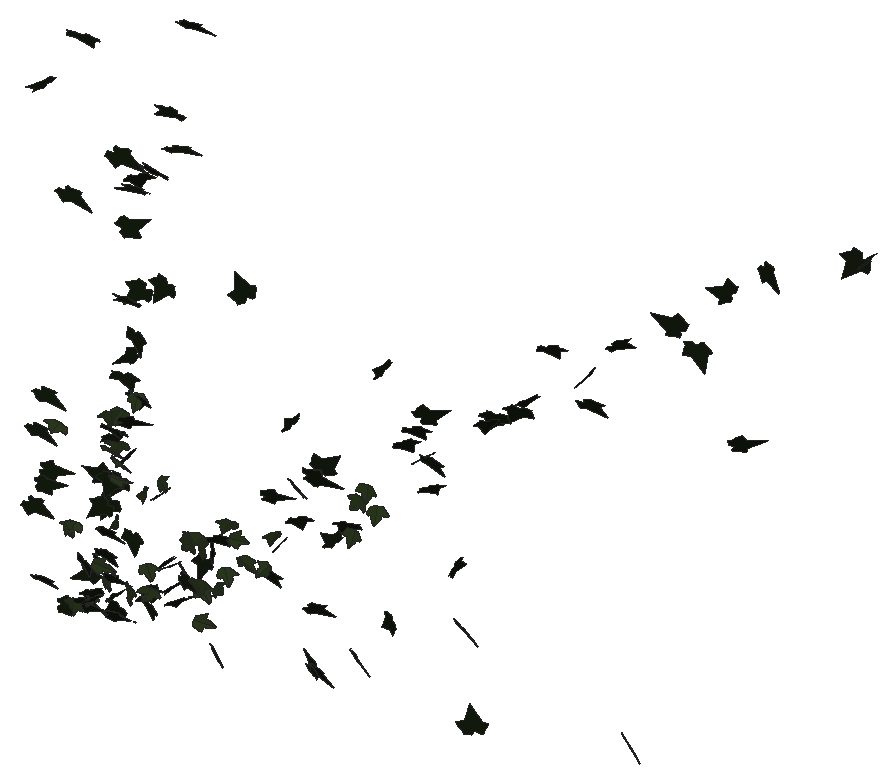
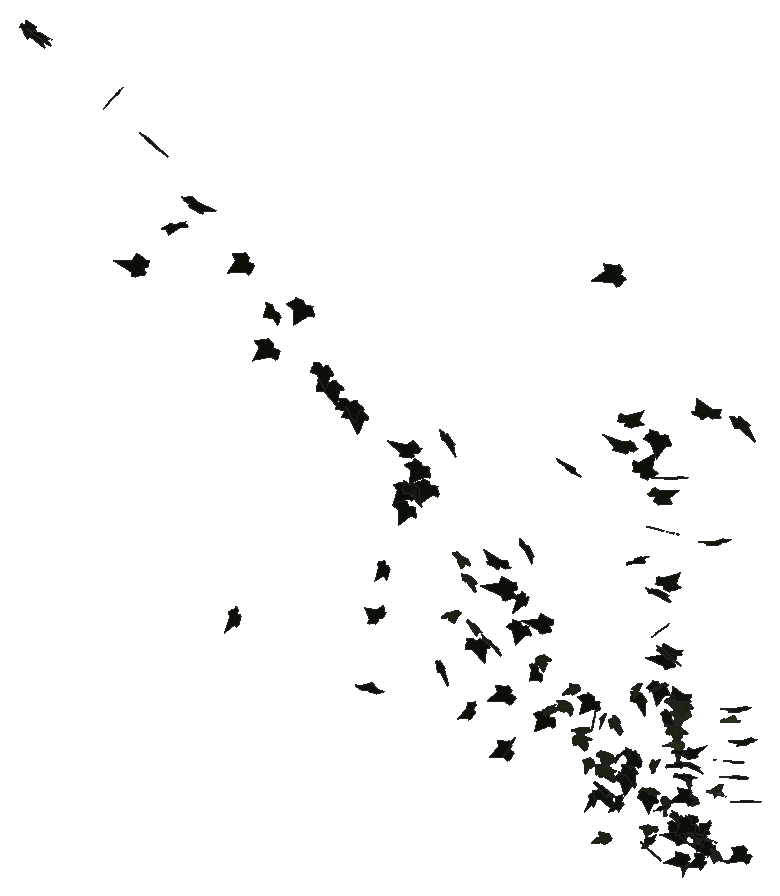
# SketchUp Ruby script. Lengths in inches.
U = 1.inch
M = Sketchup.active_model
def pt(a) = Geom::Point3d.new(a.map { |v| v * U })
def face(e, loops, mat)
  f = e.add_face(loops[0].map { |a| pt(a) })
  loops[1..].each { |l| e.add_face(l.map { |a| pt(a) }).erase! }
  f.material = f.back_material = mat if mat
  f
end
# faces: each face lists its corners as indices into pts; further lists are holes
def faces(e, pts, list, mat = nil) = list.each { |f| face(e, (f[0].is_a?(Array) ? f : [f]).map { |l| l.map { |i| pts[i] } }, mat) }
# xy, xz, yz: faces in a plane at the given z, y or x. An outline is a flat list of corners, or four numbers for a rectangle; further outlines are holes
def ring(l) = l.size == 4 ? [[l[0], l[1]], [l[2], l[1]], [l[2], l[3]], [l[0], l[3]]] : l.each_slice(2).to_a
def flat(e, list, mat, &to3) = list.each { |f| face(e, (f[0].is_a?(Array) ? f : [f]).map { |l| ring(l).map { |u, v| to3.(u, v) } }, mat) }
def xy(e, z, list, mat = nil) = flat(e, list, mat) { |x, y| [x, y, z] }
def xz(e, y, list, mat = nil) = flat(e, list, mat) { |x, z| [x, y, z] }
def yz(e, x, list, mat = nil) = flat(e, list, mat) { |y, z| [x, y, z] }
def lines(e, pts, list) = list.each { |a, b| e.add_line(pt(pts[a]), pt(pts[b])) }
# prism: a flat outline (further loops are holes) pulled along v
def prism(e, loops, v, mat = nil)
  f = face(e, loops, mat); d = Geom::Vector3d.new(v.map { |x| x * U })
  f.pushpull(f.normal.samedirection?(d) ? d.length : -d.length)
end
def box(e, o, s, mat = nil) = prism(e, [[o, [o[0] + s[0], o[1], o[2]], [o[0] + s[0], o[1] + s[1], o[2]], [o[0], o[1] + s[1], o[2]]]], [0, 0, s[2]], mat)
def at(x, y, z, deg = 0) = Geom::Transformation.translation(pt([x, y, z])) * Geom::Transformation.rotation(ORIGIN, Z_AXIS, deg.degrees)
def axes(o, x, y, z) = Geom::Transformation.new([*x, 0, *y, 0, *z, 0, *pt(o).to_a, 1])
def part(name) = M.definitions.add(name)
# library, detail: a bought-in or finely detailed component or shape, given as its bounding box
def library(name, o, s) = part(name).tap { |d| box(d.entities, o, s) }
def detail(e, o, s) = box(e.add_group.entities, o, s)
def put(e, d, t, mat = nil) = e.add_instance(d, t).tap { |i| i.material = mat if mat }
def group(e, t, mat = nil) = e.add_group.tap { |g| g.transformation = t; g.material = mat if mat }.entities
root = M.entities
M.materials.add("1026 AP 7946 SUNNY SIDE UP").color = [254, 231, 186]
M.materials.add("efeu1").color = [18, 25, 13]
M.materials.add("efeu2").color = [43, 57, 29]
c1 = part("ivyleaf_9")
p = [[1.54,2.16,1.25],[1.36,2.04,1.19],[-0.21,0.99,0.68],[-0.71,1.11,0.82],[-0.85,0.86,0.67],[-0.8,0.17,0.21],
  [-0.9,-0.01,0.1],[-0.67,-0.16,-0.02],[-0.08,-0.08,-0.05],[-0.03,-0.6,-0.4],[0.65,-0.88,-0.66],[0.83,-0.6,-0.49],
  [1.29,-0.42,-0.43],[1.8125,-0.07,-0.26],[1.21,0.44,0.15]]
faces(c1.entities,p,[[0,1,2,3,4,5,6,7,8,9,10,11,12,13,14]],"efeu1")
c2 = part("ivyleaf_10")
p = [[0,0.5,-0.03],[-0.0625,2.02,-0.43],[-0.19,2.01,-0.46],[-0.54,1.05,-0.29],[-0.52,0.625,-0.18],[-0.83,0.76,-0.28],
  [-1.16,0.64,-0.33],[-1.15,0.33,-0.24],[-0.77,-0.39,0.02],[-0.3,-0.51,0.16],[0.04,-0.48,0.23],[-0.02,2.01,-0.4375],
  [-0.06,2.01,-0.43],[0.04,-0.49,0.23],[0.67,-0.49,0.14],[1.38,0.36,-0.2],[1.375,0.51,-0.24],[0.81,0.65,-0.19],
  [0.62,0.59,-0.15],[0.6,1.09,-0.28],[0.5,1.23,-0.31]]
faces(c2.entities,p,[[0,1,2,3,4,5,6,7,8,9,10],[11,12,0,13,14,15,16,17,18,19,20]],"efeu2")
put(root,c1,axes([142.13,213.74,300.73],[0.26757,-0.36179,-0.03573],[0.28317,0.11532,-0.34897],[0.49606,0.12932,0.21848]),"1026 AP 7946 SUNNY SIDE UP")
put(root,c1,axes([142.21,213.26,296.25],[0.25217,-0.28686,-0.20351],[0.26459,0.25293,-0.23814],[0.47785,0.01133,0.23925]),"1026 AP 7946 SUNNY SIDE UP")
put(root,c1,axes([142.55,213.89,303.02],[0.2721,-0.36257,-0.07854],[0.28692,0.15483,-0.3402],[0.50626,0.10712,0.23502]),"1026 AP 7946 SUNNY SIDE UP")
put(root,c1,axes([143.6,212.82,323.1],[-0.30014,0.4161,-0.00083],[-0.15211,-0.04776,-0.45862],[-0.63636,-0.18483,0.11001]),"1026 AP 7946 SUNNY SIDE UP")
put(root,c1,axes([142.91,213.24,297.6875],[0.56697,-0.08892,-0.10895],[0.07634,0.35795,-0.13808],[0.20276,0.11386,0.35665]),"1026 AP 7946 SUNNY SIDE UP")
put(root,c1,axes([143.02,212.92,292.01],[0.57279,0.05558,0.03809],[0.04914,0.03732,-0.37797],[-0.09244,0.36421,0.03512]),"1026 AP 7946 SUNNY SIDE UP")
put(root,c1,axes([143.26,213.28,298.71],[0.52552,-0.15164,-0.13523],[0.16581,0.34939,-0.1381],[0.26723,0.08143,0.35163]),"1026 AP 7946 SUNNY SIDE UP")
put(root,c1,axes([143.35,215,315.34],[0.3006,-0.40103,-0.08401],[0.31703,0.16863,-0.37692],[0.55916,0.11998,0.25887]),"1026 AP 7946 SUNNY SIDE UP")
put(root,c2,axes([143.95,213.52,301.57],[-0.57814,-0.03727,0.14265],[0.09812,-0.3848,0.06166],[0.20337,0.07971,0.37579]),"1026 AP 7946 SUNNY SIDE UP")
put(root,c1,axes([143.67,215.91,324.83],[-0.14503,-0.44357,0.16843],[0.58827,-0.17195,-0.26016],[0.45665,0.08063,0.38864]),"1026 AP 7946 SUNNY SIDE UP")
put(root,c2,axes([145.16,213.34,295.85],[-0.58487,-0.02098,0.02789],[0.0317,-0.37281,-0.01438],[0.04372,-0.01033,0.38354]),"1026 AP 7946 SUNNY SIDE UP")
put(root,c1,axes([144.73,212.91,290.9],[0.482,-0.11848,-0.13664],[0.18023,0.33344,-0.03218],[0.2128,-0.01403,0.33675]),"1026 AP 7946 SUNNY SIDE UP")
put(root,c2,axes([145.17,212.77,296],[0.02609,0.34765,0.15016],[-0.02501,0.14444,-0.35705],[-0.59102,0.00923,0.02174]),"1026 AP 7946 SUNNY SIDE UP")
put(root,c2,axes([145.51,212.9375,291.24],[-0.5409,0.08491,0.02844],[-0.07609,-0.08708,-0.35191],[-0.1177,-0.33389,0.0968]),"1026 AP 7946 SUNNY SIDE UP")
put(root,c2,axes([145.48,215.72,291.48],[-0.0806,0.3404,0.08762],[-0.02401,0.08176,-0.35414],[-0.55045,-0.05341,0.00262]),"1026 AP 7946 SUNNY SIDE UP")
put(root,c1,axes([145.41,213.96,293.37],[0.07728,-0.28574,0.22088],[0.10214,-0.20733,-0.29895],[0.55391,0.0781,0.02431]),"1026 AP 7946 SUNNY SIDE UP")
put(root,c1,axes([146.0625,214.07,292.79],[-0.52562,-0.00777,0.13629],[-0.19892,-0.08855,-0.33509],[0.06227,-0.34845,0.07994]),"1026 AP 7946 SUNNY SIDE UP")
put(root,c1,axes([145.54,214.09,291.15],[0.50262,-0.15057,0.00946],[-0.00118,-0.02509,-0.36338],[0.23727,0.31882,-0.02184]),"1026 AP 7946 SUNNY SIDE UP")
put(root,c1,axes([146.21,214.54,298.73],[-0.06225,0.05881,0.38686],[-0.51416,-0.19713,-0.00487],[0.3037,-0.32168,0.07106]),"1026 AP 7946 SUNNY SIDE UP")
put(root,c1,axes([145.625,215.66,291.73],[0.4648,0.00358,0.20448],[0.31179,0.011,-0.30439],[-0.01432,0.35587,0.00943]),"1026 AP 7946 SUNNY SIDE UP")
put(root,c2,axes([146.38,214.58,296.91],[0.33826,-0.26938,-0.15687],[-0.11986,0.13169,-0.35373],[0.47035,0.22728,0.02268]),"1026 AP 7946 SUNNY SIDE UP")
put(root,c1,axes([146.06,214.69,293.88],[0.56469,0.0455,-0.01392],[-0.01436,-0.03694,-0.37135],[-0.07336,0.35749,-0.03445]),"1026 AP 7946 SUNNY SIDE UP")
put(root,c1,axes([145.88,212.94,291.27],[0.26541,-0.01318,0.32018],[0.46806,-0.09615,-0.17126],[0.14247,0.34043,-0.03382]),"1026 AP 7946 SUNNY SIDE UP")
put(root,c2,axes([146.45,215.02,302.5],[-0.38529,-0.3118,-0.00092],[0.03074,-0.01648,-0.40779],[0.48932,-0.24448,0.02489]),"1026 AP 7946 SUNNY SIDE UP")
put(root,c1,axes([146.08,214.21,293.68],[0.45152,-0.18717,0.12069],[0.14043,-0.07922,-0.35316],[0.31851,0.30026,-0.01538]),"1026 AP 7946 SUNNY SIDE UP")
put(root,c2,axes([146.51,213.33,291.98],[0.11829,0.24906,-0.2537],[-0.12127,-0.23541,-0.26937],[-0.53883,0.10766,0.00493]),"1026 AP 7946 SUNNY SIDE UP")
put(root,c1,axes([146.63,214.72,297.21],[-0.44676,-0.24461,-0.03164],[0.06783,-0.00532,-0.38485],[0.38139,-0.28559,0.03137]),"1026 AP 7946 SUNNY SIDE UP")
put(root,c1,axes([146.72,212.8,291.95],[0.15829,0.33526,0.06533],[0.03271,0.05798,-0.36026],[-0.53497,0.10274,-0.0027]),"1026 AP 7946 SUNNY SIDE UP")
put(root,c1,axes([146.8,212.85,292.49],[0.14779,0.31622,-0.14973],[-0.05778,-0.14256,-0.34065],[-0.54537,0.1008,-0.00448]),"1026 AP 7946 SUNNY SIDE UP")
put(root,c2,axes([146.83,215.21,300.66],[-0.51905,-0.19331,0.07779],[-0.07471,-0.0698,-0.3928],[0.3183,-0.33161,0.03465]),"1026 AP 7946 SUNNY SIDE UP")
put(root,c1,axes([146.71,215.46,298.3],[-0.32785,-0.30649,0.08122],[-0.02057,-0.08805,-0.38041],[0.49788,-0.20546,0.03777]),"1026 AP 7946 SUNNY SIDE UP")
put(root,c1,axes([147.03,213.82,297.5],[-0.57913,-0.08341,0.03255],[-0.02998,-0.05955,-0.38544],[0.13728,-0.36488,0.05316]),"1026 AP 7946 SUNNY SIDE UP")
put(root,c1,axes([146.43,214.26,295.55],[0.55766,0.00088,0.10681],[0.16301,-0.00736,-0.36533],[0.00193,0.36942,-0.00537]),"1026 AP 7946 SUNNY SIDE UP")
put(root,c1,axes([146.89,214.59,298.79],[-0.42628,-0.26742,-0.027],[0.08186,-0.01791,-0.38912],[0.41428,-0.27163,0.0491]),"1026 AP 7946 SUNNY SIDE UP")
put(root,c2,axes([146.98,215.28,302.6],[0.60749,-0.0607,-0.07054],[-0.11257,-0.01786,-0.40194],[0.08896,0.3919,-0.02689]),"1026 AP 7946 SUNNY SIDE UP")
put(root,c1,axes([147.57,215.68,306.33],[-0.5662,0.18275,-0.07188],[0.01148,-0.13552,-0.39932],[-0.30796,-0.34104,0.11728]),"1026 AP 7946 SUNNY SIDE UP")
put(root,c1,axes([146.72,215.1,318.87],[0.36025,-0.35595,-0.19957],[0.30419,0.29,-0.31485],[0.55821,0.07169,0.30038]),"1026 AP 7946 SUNNY SIDE UP")
put(root,c2,axes([147.01,214.03,300.95],[-0.13961,-0.33774,0.1794],[0.59888,-0.07814,0.04299],[-0.00196,0.18103,0.35819]),"1026 AP 7946 SUNNY SIDE UP")
put(root,c1,axes([147.25,214.18,302.17],[-0.15527,-0.32678,0.2033],[0.43444,-0.20322,-0.20354],[0.41641,0.09018,0.28816]),"1026 AP 7946 SUNNY SIDE UP")
put(root,c1,axes([147.65,215.7,303.6875],[0.505,0.09081,-0.22566],[-0.33683,-0.04905,-0.34399],[-0.16164,0.38594,0.0118]),"1026 AP 7946 SUNNY SIDE UP")
put(root,c1,axes([147.29,214.0625,301.91],[-0.14049,-0.37426,-0.09172],[0.60408,-0.08564,-0.02745],[0.00935,-0.09056,0.39495]),"1026 AP 7946 SUNNY SIDE UP")
put(root,c2,axes([147.23,214.26,299.04],[0.39017,-0.29292,-0.00677],[0.46063,0.24816,0.00152],[0.00491,-0.00379,0.39546]),"1026 AP 7946 SUNNY SIDE UP")
put(root,c2,axes([147.23,212.79,294.34],[0.11746,0.09075,0.36258],[0.46144,0.19605,-0.11527],[-0.33587,0.30109,-0.03156]),"1026 AP 7946 SUNNY SIDE UP")
put(root,c1,axes([147.52,215.5625,295.02],[-0.05434,-0.37089,0.0083],[0.00994,-0.01079,-0.38373],[0.58332,-0.03437,0.00731]),"1026 AP 7946 SUNNY SIDE UP")
put(root,c2,axes([147.67,215.69,303.68],[0.30586,0.32762,-0.12208],[-0.07216,-0.11258,-0.39278],[-0.54406,0.19912,-0.01653]),"1026 AP 7946 SUNNY SIDE UP")
put(root,c1,axes([147.4375,214.87,314.5625],[0.68626,-0.00428,-0.0369],[0.00386,0.43735,-0.02045],[0.05656,0.02205,0.44918]),"1026 AP 7946 SUNNY SIDE UP")
put(root,c1,axes([148.08,215.8125,310.54],[-0.64583,-0.10068,0.00761],[0.00253,-0.03986,-0.43402],[0.15879,-0.40886,0.03788]),"1026 AP 7946 SUNNY SIDE UP")
put(root,c1,axes([147.71,215.56,307.68],[0.06917,-0.40537,0.06744],[0.01051,-0.06744,-0.42045],[0.64616,0.04449,-0.00038]),"1026 AP 7946 SUNNY SIDE UP")
put(root,c2,axes([147.53,214.01,300.42],[0.23363,-0.34168,0.11434],[0.53731,0.09565,-0.16446],[0.17743,0.16025,0.34749]),"1026 AP 7946 SUNNY SIDE UP")
put(root,c1,axes([148.28,215.28,317.02],[-0.69912,-0.0324,0.02889],[0.03677,-0.4286,-0.12988],[0.05669,-0.12159,0.44053]),"1026 AP 7946 SUNNY SIDE UP")
put(root,c1,axes([148.29,214.32,300.87],[-0.31592,0.30495,-0.14464],[0.10863,-0.12463,-0.3768],[-0.51776,-0.21222,0.0092]),"1026 AP 7946 SUNNY SIDE UP")
put(root,c2,axes([148.11,215.875,297.73],[-0.00167,-0.09132,-0.38407],[-0.09676,-0.36743,0.09088],[-0.59494,0.06001,-0.0137]),"1026 AP 7946 SUNNY SIDE UP")
put(root,c1,axes([147.77,214.5,305.61],[-0.1584,-0.39345,0.0301],[0.44273,-0.09438,-0.28781],[0.43494,-0.04722,0.30393]),"1026 AP 7946 SUNNY SIDE UP")
put(root,c1,axes([148.23,214.55,310.35],[-0.61807,-0.11805,0.13463],[0.14467,-0.41046,-0.09878],[0.23703,-0.05729,0.41134]),"1026 AP 7946 SUNNY SIDE UP")
put(root,c1,axes([148.45,212.81,292.72],[0.03564,0.32841,0.14947],[-0.06939,0.14498,-0.33442],[-0.55907,0.00294,0.05104]),"1026 AP 7946 SUNNY SIDE UP")
put(root,c1,axes([148.66,212.85,292.15],[0.14263,0.109,-0.33838],[-0.50261,-0.10535,-0.12734],[-0.21097,0.32469,0.0746]),"1026 AP 7946 SUNNY SIDE UP")
put(root,c2,axes([148.48,212.81,297.49],[0.02598,-0.34295,-0.16815],[0.05765,0.16212,-0.35033],[0.59311,-0.00074,0.04142]),"1026 AP 7946 SUNNY SIDE UP")
put(root,c1,axes([148.06,212.89,291.39],[0.38477,-0.03013,0.26411],[0.40563,0.01044,-0.25216],[0.02077,0.35437,0.03198]),"1026 AP 7946 SUNNY SIDE UP")
put(root,c2,axes([148.36,215.73,293.24],[0.35973,0.2633,0.09191],[0.098,0.06203,-0.35892],[-0.42524,0.23704,-0.00497]),"1026 AP 7946 SUNNY SIDE UP")
put(root,c1,axes([148.88,215.75,291.82],[-0.52233,0.16557,-0.01158],[-0.00642,-0.0354,-0.38102],[-0.26097,-0.33052,0.03256]),"1026 AP 7946 SUNNY SIDE UP")
put(root,c2,axes([149.42,212.89,293.59],[-0.44225,0.22386,0.0394],[-0.08397,-0.00807,-0.36814],[-0.34675,-0.28356,0.0389]),"1026 AP 7946 SUNNY SIDE UP")
put(root,c1,axes([149.125,214.97,291.5],[0.02887,-0.28627,0.23942],[0.10007,-0.22837,-0.29426],[0.57272,0.05434,0.03935]),"1026 AP 7946 SUNNY SIDE UP")
put(root,c1,axes([149.51,215.28,318.44],[-0.65879,-0.05655,0.17966],[0.15439,-0.43676,0.09438],[0.24401,0.12368,0.42533]),"1026 AP 7946 SUNNY SIDE UP")
put(root,c2,axes([149.5,212.85,292.8125],[-0.22565,0.31461,-0.11034],[-0.0409,0.10762,0.35626],[0.52188,0.14446,-0.01979]),"1026 AP 7946 SUNNY SIDE UP")
put(root,c1,axes([149.04,212.86,303.82],[0.35755,0.02717,0.33647],[0.49335,0.09616,-0.23283],[-0.14805,0.38605,0.03672]),"1026 AP 7946 SUNNY SIDE UP")
put(root,c1,axes([150.11,216.03,322.15],[-0.66051,-0.13232,0.14026],[0.12435,-0.42291,-0.17361],[0.27233,-0.12783,0.41945]),"1026 AP 7946 SUNNY SIDE UP")
put(root,c1,axes([150.05,212.73,319.62],[0.34936,0.38364,-0.07795],[-0.02823,-0.07943,-0.45652],[-0.61489,0.22162,-0.02333]),"1026 AP 7946 SUNNY SIDE UP")
put(root,c1,axes([150.08,215.25,311.77],[-0.32085,-0.35384,0.14706],[-0.09635,-0.1317,-0.42138],[0.59336,-0.21271,0.0111]),"1026 AP 7946 SUNNY SIDE UP")
put(root,c1,axes([150.66,213.08,293.6],[0.14802,0.35034,-0.01896],[-0.00149,-0.02086,-0.37381],[-0.55181,0.09403,-0.00408]),"1026 AP 7946 SUNNY SIDE UP")
put(root,c2,axes([150.77,212.91,293.85],[0.4989,0.1519,-0.09819],[-0.18184,0.02306,-0.35538],[-0.21646,0.33074,0.07222]),"1026 AP 7946 SUNNY SIDE UP")
put(root,c1,axes([150.17,215.88,320.07],[0.27266,-0.39579,0.14288],[0.62744,0.10743,-0.19434],[0.20676,0.19594,0.40134]),"1026 AP 7946 SUNNY SIDE UP")
put(root,c1,axes([150.88,215.63,294.18],[0.48571,-0.22211,-0.07244],[-0.11721,0.01422,-0.39052],[0.34644,0.3162,-0.03056]),"1026 AP 7946 SUNNY SIDE UP")
put(root,c1,axes([151.71,212.82,300.33],[-0.08927,0.38447,-0.03207],[-0.00154,-0.03381,-0.40053],[-0.60681,-0.05647,0.00573]),"1026 AP 7946 SUNNY SIDE UP")
put(root,c2,axes([151.9375,215.96,296.23],[-0.43172,-0.12644,0.23239],[-0.26177,-0.16667,-0.30499],[0.31244,-0.31435,0.06558]),"1026 AP 7946 SUNNY SIDE UP")
put(root,c2,axes([151.67,212.83,301.04],[-0.03083,0.35089,0.18249],[-0.0822,0.17146,-0.35891],[-0.61115,-0.04077,0.03907]),"1026 AP 7946 SUNNY SIDE UP")
put(root,c1,axes([151.73,212.91,295.85],[0.22498,0.20165,0.28428],[0.16517,0.25744,-0.24945],[-0.50986,0.17237,0.04463]),"1026 AP 7946 SUNNY SIDE UP")
put(root,c1,axes([152.17,212.78,295.93],[0.1638,0.34148,0.10034],[-0.02334,0.1036,-0.36452],[-0.55704,0.09607,0.04478]),"1026 AP 7946 SUNNY SIDE UP")
put(root,c1,axes([152.26,215.94,294.95],[-0.50344,-0.03269,-0.21292],[0.32749,-0.017,-0.33001],[0.02862,-0.38061,0.03078]),"1026 AP 7946 SUNNY SIDE UP")
put(root,c2,axes([152.01,215.65,291.1875],[0.07795,0.15945,0.37357],[0.25455,0.32439,-0.16827],[-0.56706,0.16754,-0.02418]),"1026 AP 7946 SUNNY SIDE UP")
put(root,c1,axes([152.51,212.78,294.78],[-0.07539,0.36055,-0.06534],[0.01296,-0.06496,-0.37509],[-0.57606,-0.04865,0.00011]),"1026 AP 7946 SUNNY SIDE UP")
put(root,c1,axes([152.73,212.71,293.99],[0.17973,0.35375,0.00817],[-0.00394,0.00703,-0.38291],[-0.5563,0.11424,0.00535]),"1026 AP 7946 SUNNY SIDE UP")
put(root,c1,axes([153.13,214.625,293.61],[-0.00391,0.35208,-0.11368],[-0.23506,-0.1037,-0.33201],[-0.53144,0.04328,0.14769]),"1026 AP 7946 SUNNY SIDE UP")
put(root,c2,axes([153.52,212.89,298.01],[0.2085,-0.19752,-0.29952],[-0.30681,0.21567,-0.24229],[0.45795,0.23442,-0.02596]),"1026 AP 7946 SUNNY SIDE UP")
put(root,c2,axes([153.67,212.83,297.81],[-0.39205,0.11422,0.27111],[-0.41709,0.0388,-0.27671],[-0.16935,-0.35997,0.05386]),"1026 AP 7946 SUNNY SIDE UP")
put(root,c1,axes([153.14,212.89,295.53],[0.35779,-0.22206,-0.19762],[-0.1408,0.17698,-0.32157],[0.43804,0.23826,0.05805]),"1026 AP 7946 SUNNY SIDE UP")
put(root,c1,axes([153.27,212.87,330.28],[0.68517,0.02398,0.18546],[0.27196,0.08681,-0.44302],[-0.0864,0.46335,0.07621]),"1026 AP 7946 SUNNY SIDE UP")
put(root,c2,axes([153.95,215.97,297.86],[-0.38706,-0.23927,0.15503],[-0.14504,-0.12252,-0.35367],[0.42132,-0.26199,0.02067]),"1026 AP 7946 SUNNY SIDE UP")
put(root,c2,axes([153.99,213.2,295.42],[-0.5778,-0.03284,-0.02853],[0.04799,-0.03402,-0.3784],[0.04727,-0.36692,0.03545]),"1026 AP 7946 SUNNY SIDE UP")
put(root,c2,axes([153.86,213.57,294.75],[0.36111,0.23908,0.17183],[0.22107,0.09321,-0.33929],[-0.40015,0.26725,-0.03238]),"1026 AP 7946 SUNNY SIDE UP")
put(root,c2,axes([154.49,212.8,297.83],[-0.12779,0.31032,0.21063],[-0.13091,0.18693,-0.32811],[-0.56793,-0.11291,0.02824]),"1026 AP 7946 SUNNY SIDE UP")
put(root,c2,axes([154.72,213.89,294.98],[0.09169,0.26279,0.26766],[-0.11713,0.26455,-0.25837],[-0.56746,-0.01214,0.09658]),"1026 AP 7946 SUNNY SIDE UP")
put(root,c1,axes([155.125,212.92,297.93],[0.15125,-0.03982,-0.37426],[-0.47063,0.20657,-0.10382],[0.32913,0.31368,0.02353]),"1026 AP 7946 SUNNY SIDE UP")
put(root,c1,axes([155.24,212.9,291.76],[0.44467,-0.19058,-0.17868],[-0.25802,0.06331,-0.34909],[0.31095,0.32508,-0.03414]),"1026 AP 7946 SUNNY SIDE UP")
put(root,c1,axes([155.3,212.92,298.76],[0.45139,0.23821,0.07515],[0.09827,0.03674,-0.3839],[-0.37857,0.29357,-0.01005]),"1026 AP 7946 SUNNY SIDE UP")
put(root,c2,axes([155.81,213.27,296.67],[0.33915,0.30544,0.03563],[0.07466,0.00651,-0.38348],[-0.47723,0.21808,-0.03468]),"1026 AP 7946 SUNNY SIDE UP")
put(root,c2,axes([156.65,212.93,299.16],[0.03395,0.13989,0.36598],[0.14742,0.34216,-0.143],[-0.58077,0.09503,-0.01491]),"1026 AP 7946 SUNNY SIDE UP")
put(root,c1,axes([157.6875,212.73,314.81],[-0.6941,0.06679,-0.16993],[-0.24966,0.05364,0.45937],[0.1276,0.46831,-0.02555]),"1026 AP 7946 SUNNY SIDE UP")
put(root,c2,axes([157.12,213.24,297.89],[-0.43655,0.02238,-0.26369],[0.38272,-0.09836,-0.28128],[-0.13002,-0.36467,0.05739]),"1026 AP 7946 SUNNY SIDE UP")
put(root,c2,axes([158.18,213.89,297.49],[-0.17235,-0.12163,0.3553],[0.05666,-0.36254,-0.1218],[0.57327,-0.00073,0.11886]),"1026 AP 7946 SUNNY SIDE UP")
put(root,c1,axes([158.04,214.02,297.05],[0.57895,0.09959,-0.02922],[-0.03363,-0.03149,-0.3923],[-0.15956,0.36798,-0.02334]),"1026 AP 7946 SUNNY SIDE UP")
put(root,c2,axes([159.41,213.04,300.375],[-0.19424,-0.36314,0.03924],[-0.00967,-0.04031,-0.39533],[0.5744,-0.12348,0.00662]),"1026 AP 7946 SUNNY SIDE UP")
put(root,c1,axes([159.5,213.23,299.53],[0.12627,0.22762,0.31022],[0.11366,0.29155,-0.24625],[-0.58091,0.10652,0.01925]),"1026 AP 7946 SUNNY SIDE UP")
put(root,c1,axes([159.125,212.74,302.78],[0.30803,0.03285,0.35725],[0.54099,0.04253,-0.20424],[-0.08369,0.39585,-0.00534]),"1026 AP 7946 SUNNY SIDE UP")
put(root,c1,axes([160.85,212.73,307.89],[-0.10381,0.35476,0.21459],[-0.1021,0.19728,-0.36976],[-0.63715,-0.08942,0.02429]),"1026 AP 7946 SUNNY SIDE UP")
put(root,c1,axes([160.99,212.75,304.14],[0.52666,-0.07275,-0.2115],[-0.28413,0.11614,-0.34611],[0.19013,0.37507,0.06864]),"1026 AP 7946 SUNNY SIDE UP")
put(root,c1,axes([161.15,212.83,302.02],[0.35851,0.31704,-0.041],[-0.01018,-0.0465,-0.40195],[-0.50269,0.22705,-0.0211]),"1026 AP 7946 SUNNY SIDE UP")
put(root,c1,axes([162.18,213.17,292.76],[0.04434,-0.37699,0.20166],[0.04123,0.19949,0.38882],[-0.66821,-0.01271,0.03737]),"1026 AP 7946 SUNNY SIDE UP")
put(root,c1,axes([161.65,213.31,304.66],[0.49105,-0.01326,0.3676],[0.5485,-0.09037,-0.31844],[0.12046,0.46555,-0.04851]),"1026 AP 7946 SUNNY SIDE UP")
put(root,c1,axes([161.99,213.08,292.94],[0.63966,-0.11607,0.05514],[0.06236,-0.05742,-0.43379],[0.19153,0.40636,-0.04292]),"1026 AP 7946 SUNNY SIDE UP")
put(root,c1,axes([162.12,212.85,296.82],[0.50128,0.1524,0.19542],[0.295,0.04293,-0.36175],[-0.24199,0.36803,-0.03618]),"1026 AP 7946 SUNNY SIDE UP")
put(root,c1,axes([162.93,213.86,300.79],[-0.15041,0.31151,0.23126],[-0.25493,0.17503,-0.32291],[-0.5455,-0.16769,0.08714]),"1026 AP 7946 SUNNY SIDE UP")
put(root,c1,axes([162.86,215.14,301.3],[0.20763,0.30972,-0.21353],[-0.24095,-0.15732,-0.34077],[-0.53586,0.19074,0.07049]),"1026 AP 7946 SUNNY SIDE UP")
put(root,c1,axes([162.92,212.8125,305.83],[-0.2995,0.1027,0.35513],[0.51979,-0.10211,0.21929],[0.22071,0.37985,-0.03453]),"1026 AP 7946 SUNNY SIDE UP")
put(root,c2,axes([164.1,214.03,301.65],[0.57779,-0.14721,0.04518],[0.04616,-0.0465,-0.40673],[0.23746,0.36723,-0.03087]),"1026 AP 7946 SUNNY SIDE UP")
put(root,c2,axes([164.76,215.28,302.79],[0.3723,0.31128,-0.09122],[-0.06527,-0.0818,-0.40305],[-0.50545,0.23985,-0.01514]),"1026 AP 7946 SUNNY SIDE UP")
put(root,c2,axes([165.12,213.3,304.375],[0.5269,-0.14805,-0.16476],[-0.21686,0.08108,-0.37652],[0.26408,0.36197,0.01953]),"1026 AP 7946 SUNNY SIDE UP")
put(root,c1,axes([164.88,213.1,294.8125],[0.52323,-0.27589,-0.04742],[-0.08397,0.00509,-0.4442],[0.4313,0.33568,-0.02895]),"1026 AP 7946 SUNNY SIDE UP")
put(root,c2,axes([165.83,213.05,305.5],[0.61103,-0.08585,0.06233],[0.09967,0.00449,-0.40955],[0.13223,0.39333,0.02069]),"1026 AP 7946 SUNNY SIDE UP")
put(root,c1,axes([167.2,213.51,297.46],[0.14527,-0.05439,-0.41313],[-0.63192,0.03341,-0.09993],[0.07078,0.40987,-0.04422]),"1026 AP 7946 SUNNY SIDE UP")
put(root,c1,axes([167.33,212.7,313.58],[-0.2164,0.39249,0.12763],[-0.07126,0.11302,-0.42778],[-0.64218,-0.1448,0.00446]),"1026 AP 7946 SUNNY SIDE UP")
put(root,c1,axes([168.66,212.69,309.49],[0.37859,0.33477,0.03909],[0.07345,0.01067,-0.4235],[-0.52432,0.24322,-0.0311]),"1026 AP 7946 SUNNY SIDE UP")
put(root,c1,axes([169.34,212.68,310.61],[0.51215,0.25827,-0.00357],[-0.00534,-0.00365,-0.42825],[-0.40615,0.32573,0.00113]),"1026 AP 7946 SUNNY SIDE UP")
put(root,c1,axes([170.12,212.82,309.04],[-0.1452,0.39797,-0.07297],[-0.06864,-0.08433,-0.41671],[-0.63252,-0.0822,0.06197]),"1026 AP 7946 SUNNY SIDE UP")
put(root,c1,axes([170.14,213.02,308.86],[0.646,0.0167,-0.04337],[-0.0633,-0.04338,-0.42168],[-0.03295,0.41071,-0.04035]),"1026 AP 7946 SUNNY SIDE UP")
put(root,c1,axes([170.02,212.78,311.53],[0.01277,0.04095,0.43593],[0.66634,0.03002,-0.0112],[-0.04864,0.42193,-0.039]),"1026 AP 7946 SUNNY SIDE UP")
put(root,c1,axes([170.48,212.66,307.33],[0.34062,0.35079,0.05918],[0.04678,0.04681,-0.42446],[-0.55648,0.21865,0.00054]),"1026 AP 7946 SUNNY SIDE UP")
put(root,c1,axes([171.96,213.125,302.7],[-0.06483,0.08976,-0.42647],[-0.35503,0.34787,0.10278],[0.56448,0.2291,0.01567]),"1026 AP 7946 SUNNY SIDE UP")
put(root,c1,axes([172.39,213.26,298.9375],[0.18037,-0.32907,0.29799],[0.26988,-0.24342,-0.35455],[0.63597,0.19663,0.06594]),"1026 AP 7946 SUNNY SIDE UP")
put(root,c1,axes([173.5,212.93,293.18],[-0.64484,-0.06759,0.1145],[0.16106,0.06085,0.42636],[-0.12693,0.42062,-0.0407]),"1026 AP 7946 SUNNY SIDE UP")
put(root,c1,axes([174.54,212.78,312.81],[0.24121,0.37407,-0.14381],[-0.0624,-0.1368,-0.41705],[-0.62588,0.1578,-0.01384]),"1026 AP 7946 SUNNY SIDE UP")
put(root,c1,axes([174.95,212.875,313.35],[0.35632,0.25635,-0.26242],[-0.22506,-0.21428,-0.35257],[-0.52354,0.26659,-0.02704]),"1026 AP 7946 SUNNY SIDE UP")
put(root,c1,axes([176.54,212.96,314.24],[0.298,0.2659,-0.28842],[-0.23752,-0.23778,-0.33757],[-0.56061,0.24209,-0.01029]),"1026 AP 7946 SUNNY SIDE UP")
put(root,c1,axes([177.19,212.85,315.11],[0.08061,0.42836,-0.03922],[-0.00348,-0.04053,-0.44467],[-0.67655,0.05125,-0.00239]),"1026 AP 7946 SUNNY SIDE UP")
put(root,c1,axes([178.78,212.72,318.98],[0.51636,0.29128,-0.02365],[-0.04768,-0.00287,-0.45185],[-0.45717,0.3293,0.02042]),"1026 AP 7946 SUNNY SIDE UP")
put(root,c1,axes([180.61,213.72,315.75],[0.64447,0.14078,0.06444],[0.11247,-0.019,-0.44458],[-0.21397,0.41405,-0.03961]),"1026 AP 7946 SUNNY SIDE UP")
put(root,c1,axes([181.23,212.73,317.78],[-0.28286,0.26284,-0.31775],[-0.23245,0.27338,0.32885],[0.5952,0.23168,-0.02257]),"1026 AP 7946 SUNNY SIDE UP")
put(root,c1,axes([183.27,212.9,320.65],[0.39157,0.27528,0.26005],[0.28557,0.17371,-0.38108],[-0.51129,0.30785,-0.01369]),"1026 AP 7946 SUNNY SIDE UP")
put(root,c1,axes([183.32,213.86,295.52],[0.6064,-0.21313,-0.19892],[-0.29996,0.04944,-0.45128],[0.33669,0.4279,-0.04378]),"1026 AP 7946 SUNNY SIDE UP")
put(root,c1,axes([187.82,212.83,323.25],[-0.22828,0.11667,0.43037],[-0.58322,0.19364,-0.18767],[-0.35163,-0.39692,0.03187]),"1026 AP 7946 SUNNY SIDE UP")
put(root,c1,axes([188.37,213.75,321.96],[-0.1273,-0.41669,-0.17248],[0.07569,0.15868,-0.43606],[0.70066,-0.09285,0.01577]),"1026 AP 7946 SUNNY SIDE UP")
put(root,c1,axes([191.36,212.84,326.7],[-0.41407,0.28939,0.26121],[-0.31319,0.15803,-0.4006],[-0.51564,-0.32838,0.03355]),"1026 AP 7946 SUNNY SIDE UP")
put(root,c1,axes([191.72,212.95,317.3],[0.24803,0.0219,0.45828],[0.65045,0.16736,-0.15867],[-0.25904,0.4412,0.0404]),"1026 AP 7946 SUNNY SIDE UP")
put(root,c1,axes([193.8125,212.9,329.13],[0.30256,-0.36176,-0.24281],[-0.19903,0.19709,-0.42062],[0.64724,0.22971,-0.01584]),"1026 AP 7946 SUNNY SIDE UP")
put(root,c1,axes([200.03,213.46,331.66],[-0.72737,-0.11175,-0.06156],[0.10933,-0.03758,-0.48749],[0.16602,-0.46483,0.05132]),"1026 AP 7946 SUNNY SIDE UP")
put(root,c1,axes([200.64,213.39,331.85],[-0.42392,0.35119,-0.19394],[0.068,-0.20251,-0.44944],[-0.62434,-0.26051,0.08273]),"1026 AP 7946 SUNNY SIDE UP")
